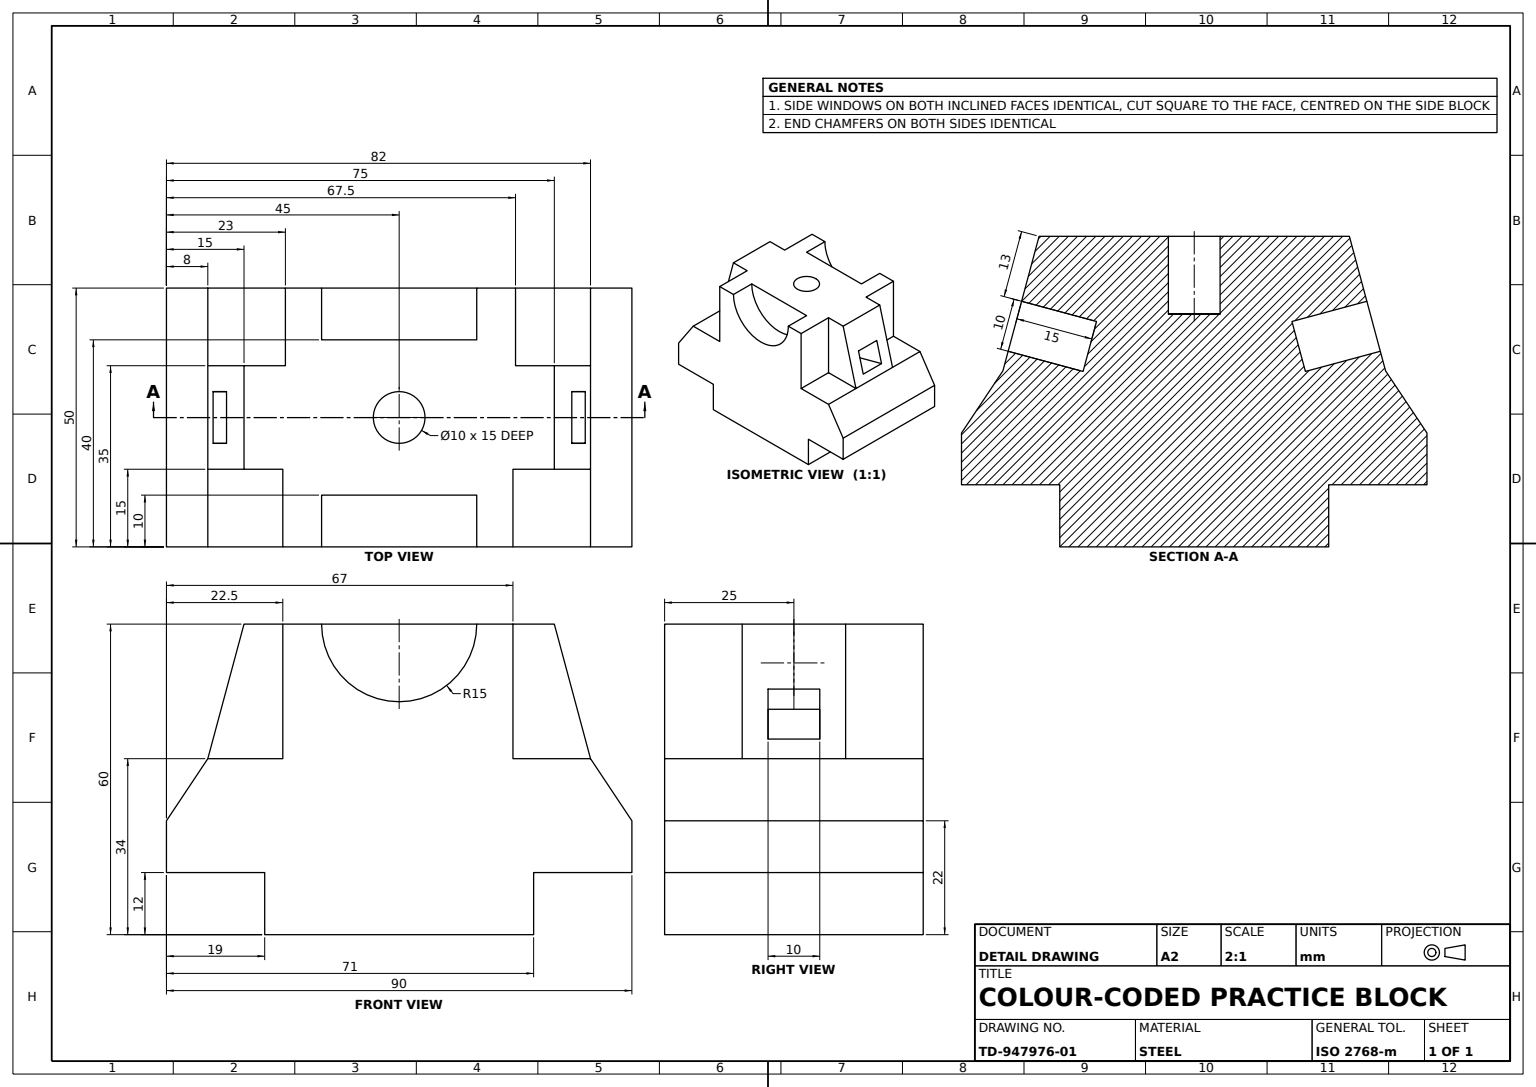
ISO-10303-21;
HEADER;
FILE_DESCRIPTION((''),'2;1');
FILE_NAME('','',(''),(''),'','','');
FILE_SCHEMA(('AUTOMOTIVE_DESIGN'));
ENDSEC;
DATA;
#1=APPLICATION_CONTEXT('');
#2=PRODUCT_CONTEXT('',#1,'mechanical');
#3=PRODUCT('','','',(#2));
#4=PRODUCT_DEFINITION_FORMATION('','',#3);
#5=PRODUCT_DEFINITION_CONTEXT('',#1,'design');
#6=PRODUCT_DEFINITION('','',#4,#5);
#7=PRODUCT_DEFINITION_SHAPE('','',#6);
#8=(LENGTH_UNIT()NAMED_UNIT(*)SI_UNIT(.MILLI.,.METRE.));
#9=(NAMED_UNIT(*)PLANE_ANGLE_UNIT()SI_UNIT($,.RADIAN.));
#10=(NAMED_UNIT(*)SI_UNIT($,.STERADIAN.)SOLID_ANGLE_UNIT());
#11=UNCERTAINTY_MEASURE_WITH_UNIT(LENGTH_MEASURE(1.E-05),#8,'distance_accuracy_value','');
#12=(GEOMETRIC_REPRESENTATION_CONTEXT(3)GLOBAL_UNCERTAINTY_ASSIGNED_CONTEXT((#11))GLOBAL_UNIT_ASSIGNED_CONTEXT((#8,#9,#10))REPRESENTATION_CONTEXT('',''));
#13=CARTESIAN_POINT('',(11.,60.,50.));
#14=VERTEX_POINT('',#13);
#15=CARTESIAN_POINT('',(41.,60.,50.));
#16=VERTEX_POINT('',#15);
#17=CARTESIAN_POINT('',(26.,60.,50.));
#18=DIRECTION('',(0.,0.,1.));
#19=DIRECTION('',(1.,0.,0.));
#20=AXIS2_PLACEMENT_3D('',#17,#18,#19);
#21=CIRCLE('',#20,15.);
#22=EDGE_CURVE('',#14,#16,#21,.T.);
#23=ORIENTED_EDGE('',*,*,#22,.F.);
#24=CARTESIAN_POINT('',(3.5,60.,50.));
#25=VERTEX_POINT('',#24);
#26=CARTESIAN_POINT('',(4.,60.,50.));
#27=DIRECTION('',(-1.,0.,0.));
#28=VECTOR('',#27,1000.);
#29=LINE('',#26,#28);
#30=EDGE_CURVE('',#14,#25,#29,.T.);
#31=ORIENTED_EDGE('',*,*,#30,.T.);
#32=CARTESIAN_POINT('',(3.5,34.,50.));
#33=VERTEX_POINT('',#32);
#34=DIRECTION('',(0.,1.,0.));
#35=VECTOR('',#34,1000.);
#36=LINE('',#24,#35);
#37=EDGE_CURVE('',#33,#25,#36,.T.);
#38=ORIENTED_EDGE('',*,*,#37,.F.);
#39=CARTESIAN_POINT('',(-11.,34.,50.));
#40=VERTEX_POINT('',#39);
#41=VECTOR('',#19,1000.);
#42=LINE('',#32,#41);
#43=EDGE_CURVE('',#40,#33,#42,.T.);
#44=ORIENTED_EDGE('',*,*,#43,.F.);
#45=CARTESIAN_POINT('',(-19.,22.,50.));
#46=VERTEX_POINT('',#45);
#47=DIRECTION('',(-0.554700196,-0.832050294,0.));
#48=VECTOR('',#47,1000.);
#49=LINE('',#39,#48);
#50=EDGE_CURVE('',#40,#46,#49,.T.);
#51=ORIENTED_EDGE('',*,*,#50,.T.);
#52=CARTESIAN_POINT('',(-19.,12.,50.));
#53=VERTEX_POINT('',#52);
#54=DIRECTION('',(0.,-1.,0.));
#55=VECTOR('',#54,1000.);
#56=LINE('',#52,#55);
#57=EDGE_CURVE('',#46,#53,#56,.T.);
#58=ORIENTED_EDGE('',*,*,#57,.T.);
#59=CARTESIAN_POINT('',(0.,12.,50.));
#60=VERTEX_POINT('',#59);
#61=LINE('',#59,#41);
#62=EDGE_CURVE('',#53,#60,#61,.T.);
#63=ORIENTED_EDGE('',*,*,#62,.T.);
#64=CARTESIAN_POINT('',(0.,0.,50.));
#65=VERTEX_POINT('',#64);
#66=LINE('',#64,#55);
#67=EDGE_CURVE('',#60,#65,#66,.T.);
#68=ORIENTED_EDGE('',*,*,#67,.T.);
#69=CARTESIAN_POINT('',(52.,0.,50.));
#70=VERTEX_POINT('',#69);
#71=LINE('',#64,#41);
#72=EDGE_CURVE('',#65,#70,#71,.T.);
#73=ORIENTED_EDGE('',*,*,#72,.T.);
#74=CARTESIAN_POINT('',(52.,12.,50.));
#75=VERTEX_POINT('',#74);
#76=LINE('',#69,#35);
#77=EDGE_CURVE('',#70,#75,#76,.T.);
#78=ORIENTED_EDGE('',*,*,#77,.T.);
#79=CARTESIAN_POINT('',(71.,12.,50.));
#80=VERTEX_POINT('',#79);
#81=LINE('',#74,#41);
#82=EDGE_CURVE('',#75,#80,#81,.T.);
#83=ORIENTED_EDGE('',*,*,#82,.T.);
#84=CARTESIAN_POINT('',(71.,22.,50.));
#85=VERTEX_POINT('',#84);
#86=LINE('',#79,#35);
#87=EDGE_CURVE('',#80,#85,#86,.T.);
#88=ORIENTED_EDGE('',*,*,#87,.T.);
#89=CARTESIAN_POINT('',(63.,34.,50.));
#90=VERTEX_POINT('',#89);
#91=DIRECTION('',(-0.554700196,0.832050294,0.));
#92=VECTOR('',#91,1000.);
#93=LINE('',#89,#92);
#94=EDGE_CURVE('',#85,#90,#93,.T.);
#95=ORIENTED_EDGE('',*,*,#94,.T.);
#96=CARTESIAN_POINT('',(48.,34.,50.));
#97=VERTEX_POINT('',#96);
#98=LINE('',#96,#28);
#99=EDGE_CURVE('',#90,#97,#98,.T.);
#100=ORIENTED_EDGE('',*,*,#99,.T.);
#101=CARTESIAN_POINT('',(48.,60.,50.));
#102=VERTEX_POINT('',#101);
#103=LINE('',#96,#35);
#104=EDGE_CURVE('',#97,#102,#103,.T.);
#105=ORIENTED_EDGE('',*,*,#104,.T.);
#106=EDGE_CURVE('',#102,#16,#29,.T.);
#107=ORIENTED_EDGE('',*,*,#106,.T.);
#108=EDGE_LOOP('',(#23,#31,#38,#44,#51,#58,#63,#68,#73,#78,#83,#88,#95,#100,#105,#107));
#109=FACE_OUTER_BOUND('',#108,.T.);
#110=AXIS2_PLACEMENT_3D('',#64,#18,#19);
#111=PLANE('',#110);
#112=ADVANCED_FACE('',(#109),#111,.T.);
#113=CARTESIAN_POINT('',(48.5,34.,0.));
#114=VERTEX_POINT('',#113);
#115=CARTESIAN_POINT('',(48.5,60.,0.));
#116=VERTEX_POINT('',#115);
#117=LINE('',#115,#35);
#118=EDGE_CURVE('',#114,#116,#117,.T.);
#119=ORIENTED_EDGE('',*,*,#118,.T.);
#120=CARTESIAN_POINT('',(48.5,60.,15.));
#121=VERTEX_POINT('',#120);
#122=CARTESIAN_POINT('',(48.5,60.,20.));
#123=DIRECTION('',(0.,0.,-1.));
#124=VECTOR('',#123,1000.);
#125=LINE('',#122,#124);
#126=EDGE_CURVE('',#121,#116,#125,.T.);
#127=ORIENTED_EDGE('',*,*,#126,.F.);
#128=CARTESIAN_POINT('',(48.5,34.,15.));
#129=VERTEX_POINT('',#128);
#130=LINE('',#128,#35);
#131=EDGE_CURVE('',#129,#121,#130,.T.);
#132=ORIENTED_EDGE('',*,*,#131,.F.);
#133=CARTESIAN_POINT('',(48.5,34.,20.));
#134=LINE('',#133,#124);
#135=EDGE_CURVE('',#129,#114,#134,.T.);
#136=ORIENTED_EDGE('',*,*,#135,.T.);
#137=EDGE_LOOP('',(#119,#127,#132,#136));
#138=FACE_OUTER_BOUND('',#137,.T.);
#139=AXIS2_PLACEMENT_3D('',#122,#27,#18);
#140=PLANE('',#139);
#141=ADVANCED_FACE('',(#138),#140,.F.);
#142=CARTESIAN_POINT('',(26.,45.,20.));
#143=VERTEX_POINT('',#142);
#144=CARTESIAN_POINT('',(26.,60.,20.));
#145=VERTEX_POINT('',#144);
#146=LINE('',#142,#35);
#147=EDGE_CURVE('',#143,#145,#146,.T.);
#148=ORIENTED_EDGE('',*,*,#147,.F.);
#149=CARTESIAN_POINT('',(26.,45.,30.));
#150=VERTEX_POINT('',#149);
#151=CARTESIAN_POINT('',(26.,45.,25.));
#152=AXIS2_PLACEMENT_3D('',#151,#34,#18);
#153=CIRCLE('',#152,5.);
#154=EDGE_CURVE('',#150,#143,#153,.T.);
#155=ORIENTED_EDGE('',*,*,#154,.F.);
#156=CARTESIAN_POINT('',(26.,60.,30.));
#157=VERTEX_POINT('',#156);
#158=LINE('',#149,#35);
#159=EDGE_CURVE('',#150,#157,#158,.T.);
#160=ORIENTED_EDGE('',*,*,#159,.T.);
#161=CARTESIAN_POINT('',(26.,60.,25.));
#162=AXIS2_PLACEMENT_3D('',#161,#34,#18);
#163=CIRCLE('',#162,5.);
#164=EDGE_CURVE('',#157,#145,#163,.T.);
#165=ORIENTED_EDGE('',*,*,#164,.T.);
#166=EDGE_LOOP('',(#148,#155,#160,#165));
#167=FACE_OUTER_BOUND('',#166,.T.);
#168=CYLINDRICAL_SURFACE('',#152,5.);
#169=ADVANCED_FACE('',(#167),#168,.F.);
#170=CARTESIAN_POINT('',(11.,60.,0.));
#171=VERTEX_POINT('',#170);
#172=CARTESIAN_POINT('',(4.,60.,0.));
#173=VERTEX_POINT('',#172);
#174=LINE('',#172,#28);
#175=EDGE_CURVE('',#171,#173,#174,.T.);
#176=ORIENTED_EDGE('',*,*,#175,.T.);
#177=CARTESIAN_POINT('',(4.,60.,15.));
#178=VERTEX_POINT('',#177);
#179=LINE('',#26,#124);
#180=EDGE_CURVE('',#178,#173,#179,.T.);
#181=ORIENTED_EDGE('',*,*,#180,.F.);
#182=CARTESIAN_POINT('',(-4.,60.,15.));
#183=VERTEX_POINT('',#182);
#184=LINE('',#177,#28);
#185=EDGE_CURVE('',#178,#183,#184,.T.);
#186=ORIENTED_EDGE('',*,*,#185,.T.);
#187=CARTESIAN_POINT('',(-4.,60.,35.));
#188=VERTEX_POINT('',#187);
#189=VECTOR('',#18,1000.);
#190=LINE('',#182,#189);
#191=EDGE_CURVE('',#183,#188,#190,.T.);
#192=ORIENTED_EDGE('',*,*,#191,.T.);
#193=CARTESIAN_POINT('',(3.5,60.,35.));
#194=VERTEX_POINT('',#193);
#195=LINE('',#187,#28);
#196=EDGE_CURVE('',#194,#188,#195,.T.);
#197=ORIENTED_EDGE('',*,*,#196,.F.);
#198=LINE('',#193,#189);
#199=EDGE_CURVE('',#194,#25,#198,.T.);
#200=ORIENTED_EDGE('',*,*,#199,.T.);
#201=ORIENTED_EDGE('',*,*,#30,.F.);
#202=CARTESIAN_POINT('',(11.,60.,40.));
#203=VERTEX_POINT('',#202);
#204=LINE('',#202,#189);
#205=EDGE_CURVE('',#203,#14,#204,.T.);
#206=ORIENTED_EDGE('',*,*,#205,.F.);
#207=CARTESIAN_POINT('',(41.,60.,40.));
#208=VERTEX_POINT('',#207);
#209=LINE('',#202,#28);
#210=EDGE_CURVE('',#208,#203,#209,.T.);
#211=ORIENTED_EDGE('',*,*,#210,.F.);
#212=LINE('',#207,#189);
#213=EDGE_CURVE('',#208,#16,#212,.T.);
#214=ORIENTED_EDGE('',*,*,#213,.T.);
#215=ORIENTED_EDGE('',*,*,#106,.F.);
#216=CARTESIAN_POINT('',(48.,60.,35.));
#217=VERTEX_POINT('',#216);
#218=LINE('',#101,#124);
#219=EDGE_CURVE('',#102,#217,#218,.T.);
#220=ORIENTED_EDGE('',*,*,#219,.T.);
#221=CARTESIAN_POINT('',(56.,60.,35.));
#222=VERTEX_POINT('',#221);
#223=LINE('',#216,#28);
#224=EDGE_CURVE('',#222,#217,#223,.T.);
#225=ORIENTED_EDGE('',*,*,#224,.F.);
#226=CARTESIAN_POINT('',(56.,60.,15.));
#227=VERTEX_POINT('',#226);
#228=CARTESIAN_POINT('',(56.,60.,30.));
#229=LINE('',#228,#124);
#230=EDGE_CURVE('',#222,#227,#229,.T.);
#231=ORIENTED_EDGE('',*,*,#230,.T.);
#232=LINE('',#120,#41);
#233=EDGE_CURVE('',#121,#227,#232,.T.);
#234=ORIENTED_EDGE('',*,*,#233,.F.);
#235=ORIENTED_EDGE('',*,*,#126,.T.);
#236=CARTESIAN_POINT('',(41.,60.,0.));
#237=VERTEX_POINT('',#236);
#238=EDGE_CURVE('',#116,#237,#174,.T.);
#239=ORIENTED_EDGE('',*,*,#238,.T.);
#240=CARTESIAN_POINT('',(41.,60.,10.));
#241=VERTEX_POINT('',#240);
#242=LINE('',#240,#124);
#243=EDGE_CURVE('',#241,#237,#242,.T.);
#244=ORIENTED_EDGE('',*,*,#243,.F.);
#245=CARTESIAN_POINT('',(11.,60.,10.));
#246=VERTEX_POINT('',#245);
#247=LINE('',#240,#41);
#248=EDGE_CURVE('',#246,#241,#247,.T.);
#249=ORIENTED_EDGE('',*,*,#248,.F.);
#250=LINE('',#245,#124);
#251=EDGE_CURVE('',#246,#171,#250,.T.);
#252=ORIENTED_EDGE('',*,*,#251,.T.);
#253=EDGE_LOOP('',(#176,#181,#186,#192,#197,#200,#201,#206,#211,#214,#215,#220,#225,#231,#234,#235,#239,#244,#249,#252));
#254=FACE_OUTER_BOUND('',#253,.T.);
#255=EDGE_CURVE('',#145,#157,#163,.T.);
#256=ORIENTED_EDGE('',*,*,#255,.F.);
#257=ORIENTED_EDGE('',*,*,#164,.F.);
#258=EDGE_LOOP('',(#256,#257));
#259=FACE_BOUND('',#258,.T.);
#260=AXIS2_PLACEMENT_3D('',#26,#54,#123);
#261=PLANE('',#260);
#262=ADVANCED_FACE('',(#254,#259),#261,.F.);
#263=ORIENTED_EDGE('',*,*,#37,.T.);
#264=ORIENTED_EDGE('',*,*,#199,.F.);
#265=CARTESIAN_POINT('',(3.5,34.,35.));
#266=VERTEX_POINT('',#265);
#267=LINE('',#193,#35);
#268=EDGE_CURVE('',#266,#194,#267,.T.);
#269=ORIENTED_EDGE('',*,*,#268,.F.);
#270=LINE('',#265,#189);
#271=EDGE_CURVE('',#266,#33,#270,.T.);
#272=ORIENTED_EDGE('',*,*,#271,.T.);
#273=EDGE_LOOP('',(#263,#264,#269,#272));
#274=FACE_OUTER_BOUND('',#273,.T.);
#275=AXIS2_PLACEMENT_3D('',#193,#19,#123);
#276=PLANE('',#275);
#277=ADVANCED_FACE('',(#274),#276,.F.);
#278=CARTESIAN_POINT('',(4.504846,33.891235,20.));
#279=VERTEX_POINT('',#278);
#280=CARTESIAN_POINT('',(4.504846,33.891235,30.));
#281=VERTEX_POINT('',#280);
#282=LINE('',#278,#189);
#283=EDGE_CURVE('',#279,#281,#282,.T.);
#284=ORIENTED_EDGE('',*,*,#283,.T.);
#285=CARTESIAN_POINT('',(7.104581,43.547393,30.));
#286=VERTEX_POINT('',#285);
#287=DIRECTION('',(0.259973473,0.965615759,0.));
#288=VECTOR('',#287,1000.);
#289=LINE('',#285,#288);
#290=EDGE_CURVE('',#281,#286,#289,.T.);
#291=ORIENTED_EDGE('',*,*,#290,.T.);
#292=CARTESIAN_POINT('',(7.104581,43.547393,20.));
#293=VERTEX_POINT('',#292);
#294=LINE('',#292,#124);
#295=EDGE_CURVE('',#286,#293,#294,.T.);
#296=ORIENTED_EDGE('',*,*,#295,.T.);
#297=DIRECTION('',(-0.259973473,-0.965615759,0.));
#298=VECTOR('',#297,1000.);
#299=LINE('',#292,#298);
#300=EDGE_CURVE('',#293,#279,#299,.T.);
#301=ORIENTED_EDGE('',*,*,#300,.T.);
#302=EDGE_LOOP('',(#284,#291,#296,#301));
#303=FACE_OUTER_BOUND('',#302,.T.);
#304=CARTESIAN_POINT('',(-4.307488,1.159708,0.));
#305=DIRECTION('',(-0.965615759,0.259973473,0.));
#306=AXIS2_PLACEMENT_3D('',#304,#305,#297);
#307=PLANE('',#306);
#308=ADVANCED_FACE('',(#303),#307,.T.);
#309=CARTESIAN_POINT('',(4.,34.,15.));
#310=VERTEX_POINT('',#309);
#311=CARTESIAN_POINT('',(4.,34.,0.));
#312=VERTEX_POINT('',#311);
#313=CARTESIAN_POINT('',(4.,34.,50.));
#314=LINE('',#313,#124);
#315=EDGE_CURVE('',#310,#312,#314,.T.);
#316=ORIENTED_EDGE('',*,*,#315,.T.);
#317=CARTESIAN_POINT('',(-11.,34.,0.));
#318=VERTEX_POINT('',#317);
#319=LINE('',#311,#28);
#320=EDGE_CURVE('',#312,#318,#319,.T.);
#321=ORIENTED_EDGE('',*,*,#320,.T.);
#322=CARTESIAN_POINT('',(-11.,34.,15.));
#323=VERTEX_POINT('',#322);
#324=LINE('',#39,#124);
#325=EDGE_CURVE('',#323,#318,#324,.T.);
#326=ORIENTED_EDGE('',*,*,#325,.F.);
#327=LINE('',#309,#41);
#328=EDGE_CURVE('',#323,#310,#327,.T.);
#329=ORIENTED_EDGE('',*,*,#328,.T.);
#330=EDGE_LOOP('',(#316,#321,#326,#329));
#331=FACE_OUTER_BOUND('',#330,.T.);
#332=AXIS2_PLACEMENT_3D('',#313,#54,#123);
#333=PLANE('',#332);
#334=ADVANCED_FACE('',(#331),#333,.F.);
#335=CARTESIAN_POINT('',(47.495154,33.891235,20.));
#336=VERTEX_POINT('',#335);
#337=CARTESIAN_POINT('',(61.97939,37.790838,20.));
#338=VERTEX_POINT('',#337);
#339=DIRECTION('',(0.965615759,0.259973473,0.));
#340=VECTOR('',#339,1000.);
#341=LINE('',#335,#340);
#342=EDGE_CURVE('',#336,#338,#341,.T.);
#343=ORIENTED_EDGE('',*,*,#342,.F.);
#344=CARTESIAN_POINT('',(47.495154,33.891235,30.));
#345=VERTEX_POINT('',#344);
#346=LINE('',#344,#124);
#347=EDGE_CURVE('',#345,#336,#346,.T.);
#348=ORIENTED_EDGE('',*,*,#347,.F.);
#349=CARTESIAN_POINT('',(61.97939,37.790838,30.));
#350=VERTEX_POINT('',#349);
#351=LINE('',#344,#340);
#352=EDGE_CURVE('',#345,#350,#351,.T.);
#353=ORIENTED_EDGE('',*,*,#352,.T.);
#354=LINE('',#349,#124);
#355=EDGE_CURVE('',#350,#338,#354,.T.);
#356=ORIENTED_EDGE('',*,*,#355,.T.);
#357=EDGE_LOOP('',(#343,#348,#353,#356));
#358=FACE_OUTER_BOUND('',#357,.T.);
#359=DIRECTION('',(0.259973473,-0.965615759,0.));
#360=AXIS2_PLACEMENT_3D('',#344,#359,#339);
#361=PLANE('',#360);
#362=ADVANCED_FACE('',(#358),#361,.F.);
#363=ORIENTED_EDGE('',*,*,#57,.F.);
#364=CARTESIAN_POINT('',(-19.,22.,0.));
#365=VERTEX_POINT('',#364);
#366=LINE('',#45,#124);
#367=EDGE_CURVE('',#46,#365,#366,.T.);
#368=ORIENTED_EDGE('',*,*,#367,.T.);
#369=CARTESIAN_POINT('',(-19.,12.,0.));
#370=VERTEX_POINT('',#369);
#371=LINE('',#369,#55);
#372=EDGE_CURVE('',#365,#370,#371,.T.);
#373=ORIENTED_EDGE('',*,*,#372,.T.);
#374=LINE('',#52,#124);
#375=EDGE_CURVE('',#53,#370,#374,.T.);
#376=ORIENTED_EDGE('',*,*,#375,.F.);
#377=EDGE_LOOP('',(#363,#368,#373,#376));
#378=FACE_OUTER_BOUND('',#377,.T.);
#379=AXIS2_PLACEMENT_3D('',#52,#19,#123);
#380=PLANE('',#379);
#381=ADVANCED_FACE('',(#378),#380,.F.);
#382=LINE('',#182,#298);
#383=EDGE_CURVE('',#183,#323,#382,.T.);
#384=ORIENTED_EDGE('',*,*,#383,.F.);
#385=ORIENTED_EDGE('',*,*,#185,.F.);
#386=LINE('',#177,#35);
#387=EDGE_CURVE('',#310,#178,#386,.T.);
#388=ORIENTED_EDGE('',*,*,#387,.F.);
#389=ORIENTED_EDGE('',*,*,#328,.F.);
#390=EDGE_LOOP('',(#384,#385,#388,#389));
#391=FACE_OUTER_BOUND('',#390,.T.);
#392=CARTESIAN_POINT('',(0.,0.,15.));
#393=AXIS2_PLACEMENT_3D('',#392,#18,#19);
#394=PLANE('',#393);
#395=ADVANCED_FACE('',(#391),#394,.F.);
#396=ORIENTED_EDGE('',*,*,#180,.T.);
#397=LINE('',#311,#55);
#398=EDGE_CURVE('',#173,#312,#397,.T.);
#399=ORIENTED_EDGE('',*,*,#398,.T.);
#400=ORIENTED_EDGE('',*,*,#315,.F.);
#401=ORIENTED_EDGE('',*,*,#387,.T.);
#402=EDGE_LOOP('',(#396,#399,#400,#401));
#403=FACE_OUTER_BOUND('',#402,.T.);
#404=AXIS2_PLACEMENT_3D('',#313,#19,#123);
#405=PLANE('',#404);
#406=ADVANCED_FACE('',(#403),#405,.F.);
#407=ORIENTED_EDGE('',*,*,#210,.T.);
#408=CARTESIAN_POINT('',(26.,60.,40.));
#409=AXIS2_PLACEMENT_3D('',#408,#18,#19);
#410=CIRCLE('',#409,15.);
#411=EDGE_CURVE('',#203,#208,#410,.T.);
#412=ORIENTED_EDGE('',*,*,#411,.T.);
#413=EDGE_LOOP('',(#407,#412));
#414=FACE_OUTER_BOUND('',#413,.T.);
#415=PLANE('',#409);
#416=ADVANCED_FACE('',(#414),#415,.T.);
#417=CARTESIAN_POINT('',(-7.379655,47.446995,20.));
#418=VERTEX_POINT('',#417);
#419=VECTOR('',#305,1000.);
#420=LINE('',#292,#419);
#421=EDGE_CURVE('',#293,#418,#420,.T.);
#422=ORIENTED_EDGE('',*,*,#421,.T.);
#423=CARTESIAN_POINT('',(-9.97939,37.790838,20.));
#424=VERTEX_POINT('',#423);
#425=LINE('',#417,#298);
#426=EDGE_CURVE('',#418,#424,#425,.T.);
#427=ORIENTED_EDGE('',*,*,#426,.T.);
#428=LINE('',#278,#419);
#429=EDGE_CURVE('',#279,#424,#428,.T.);
#430=ORIENTED_EDGE('',*,*,#429,.F.);
#431=ORIENTED_EDGE('',*,*,#300,.F.);
#432=EDGE_LOOP('',(#422,#427,#430,#431));
#433=FACE_OUTER_BOUND('',#432,.T.);
#434=AXIS2_PLACEMENT_3D('',#292,#123,#27);
#435=PLANE('',#434);
#436=ADVANCED_FACE('',(#433),#435,.F.);
#437=CARTESIAN_POINT('',(48.,34.,35.));
#438=VERTEX_POINT('',#437);
#439=CARTESIAN_POINT('',(63.,34.,35.));
#440=VERTEX_POINT('',#439);
#441=LINE('',#439,#41);
#442=EDGE_CURVE('',#438,#440,#441,.T.);
#443=ORIENTED_EDGE('',*,*,#442,.T.);
#444=DIRECTION('',(-0.259973473,0.965615759,0.));
#445=VECTOR('',#444,1000.);
#446=LINE('',#221,#445);
#447=EDGE_CURVE('',#440,#222,#446,.T.);
#448=ORIENTED_EDGE('',*,*,#447,.T.);
#449=ORIENTED_EDGE('',*,*,#224,.T.);
#450=LINE('',#437,#55);
#451=EDGE_CURVE('',#217,#438,#450,.T.);
#452=ORIENTED_EDGE('',*,*,#451,.T.);
#453=EDGE_LOOP('',(#443,#448,#449,#452));
#454=FACE_OUTER_BOUND('',#453,.T.);
#455=CARTESIAN_POINT('',(0.,0.,35.));
#456=AXIS2_PLACEMENT_3D('',#455,#123,#27);
#457=PLANE('',#456);
#458=ADVANCED_FACE('',(#454),#457,.F.);
#459=CARTESIAN_POINT('',(-9.97939,37.790838,30.));
#460=VERTEX_POINT('',#459);
#461=CARTESIAN_POINT('',(-7.379655,47.446995,30.));
#462=VERTEX_POINT('',#461);
#463=LINE('',#461,#288);
#464=EDGE_CURVE('',#460,#462,#463,.T.);
#465=ORIENTED_EDGE('',*,*,#464,.T.);
#466=LINE('',#285,#419);
#467=EDGE_CURVE('',#286,#462,#466,.T.);
#468=ORIENTED_EDGE('',*,*,#467,.F.);
#469=ORIENTED_EDGE('',*,*,#290,.F.);
#470=LINE('',#280,#419);
#471=EDGE_CURVE('',#281,#460,#470,.T.);
#472=ORIENTED_EDGE('',*,*,#471,.T.);
#473=EDGE_LOOP('',(#465,#468,#469,#472));
#474=FACE_OUTER_BOUND('',#473,.T.);
#475=AXIS2_PLACEMENT_3D('',#285,#18,#54);
#476=PLANE('',#475);
#477=ADVANCED_FACE('',(#474),#476,.F.);
#478=CARTESIAN_POINT('',(52.,12.,0.));
#479=VERTEX_POINT('',#478);
#480=LINE('',#74,#124);
#481=EDGE_CURVE('',#75,#479,#480,.T.);
#482=ORIENTED_EDGE('',*,*,#481,.T.);
#483=CARTESIAN_POINT('',(71.,12.,0.));
#484=VERTEX_POINT('',#483);
#485=LINE('',#478,#41);
#486=EDGE_CURVE('',#479,#484,#485,.T.);
#487=ORIENTED_EDGE('',*,*,#486,.T.);
#488=LINE('',#79,#124);
#489=EDGE_CURVE('',#80,#484,#488,.T.);
#490=ORIENTED_EDGE('',*,*,#489,.F.);
#491=ORIENTED_EDGE('',*,*,#82,.F.);
#492=EDGE_LOOP('',(#482,#487,#490,#491));
#493=FACE_OUTER_BOUND('',#492,.T.);
#494=AXIS2_PLACEMENT_3D('',#74,#34,#18);
#495=PLANE('',#494);
#496=ADVANCED_FACE('',(#493),#495,.F.);
#497=EDGE_CURVE('',#143,#150,#153,.T.);
#498=ORIENTED_EDGE('',*,*,#497,.T.);
#499=ORIENTED_EDGE('',*,*,#154,.T.);
#500=EDGE_LOOP('',(#498,#499));
#501=FACE_OUTER_BOUND('',#500,.T.);
#502=PLANE('',#152);
#503=ADVANCED_FACE('',(#501),#502,.T.);
#504=ORIENTED_EDGE('',*,*,#243,.T.);
#505=CARTESIAN_POINT('',(26.,60.,0.));
#506=AXIS2_PLACEMENT_3D('',#505,#123,#27);
#507=CIRCLE('',#506,15.);
#508=EDGE_CURVE('',#237,#171,#507,.T.);
#509=ORIENTED_EDGE('',*,*,#508,.T.);
#510=ORIENTED_EDGE('',*,*,#251,.F.);
#511=CARTESIAN_POINT('',(26.,60.,10.));
#512=AXIS2_PLACEMENT_3D('',#511,#123,#27);
#513=CIRCLE('',#512,15.);
#514=EDGE_CURVE('',#241,#246,#513,.T.);
#515=ORIENTED_EDGE('',*,*,#514,.F.);
#516=EDGE_LOOP('',(#504,#509,#510,#515));
#517=FACE_OUTER_BOUND('',#516,.T.);
#518=CYLINDRICAL_SURFACE('',#512,15.);
#519=ADVANCED_FACE('',(#517),#518,.F.);
#520=ORIENTED_EDGE('',*,*,#367,.F.);
#521=ORIENTED_EDGE('',*,*,#50,.F.);
#522=CARTESIAN_POINT('',(-11.,34.,35.));
#523=VERTEX_POINT('',#522);
#524=EDGE_CURVE('',#40,#523,#324,.T.);
#525=ORIENTED_EDGE('',*,*,#524,.T.);
#526=EDGE_CURVE('',#523,#323,#324,.T.);
#527=ORIENTED_EDGE('',*,*,#526,.T.);
#528=ORIENTED_EDGE('',*,*,#325,.T.);
#529=LINE('',#317,#48);
#530=EDGE_CURVE('',#318,#365,#529,.T.);
#531=ORIENTED_EDGE('',*,*,#530,.T.);
#532=EDGE_LOOP('',(#520,#521,#525,#527,#528,#531));
#533=FACE_OUTER_BOUND('',#532,.T.);
#534=DIRECTION('',(0.832050294,-0.554700196,0.));
#535=DIRECTION('',(0.554700196,0.832050294,0.));
#536=AXIS2_PLACEMENT_3D('',#39,#534,#535);
#537=PLANE('',#536);
#538=ADVANCED_FACE('',(#533),#537,.F.);
#539=ORIENTED_EDGE('',*,*,#268,.T.);
#540=ORIENTED_EDGE('',*,*,#196,.T.);
#541=LINE('',#522,#298);
#542=EDGE_CURVE('',#188,#523,#541,.T.);
#543=ORIENTED_EDGE('',*,*,#542,.T.);
#544=LINE('',#265,#41);
#545=EDGE_CURVE('',#523,#266,#544,.T.);
#546=ORIENTED_EDGE('',*,*,#545,.T.);
#547=EDGE_LOOP('',(#539,#540,#543,#546));
#548=FACE_OUTER_BOUND('',#547,.T.);
#549=ADVANCED_FACE('',(#548),#457,.F.);
#550=CARTESIAN_POINT('',(44.895419,43.547393,20.));
#551=VERTEX_POINT('',#550);
#552=LINE('',#550,#445);
#553=EDGE_CURVE('',#336,#551,#552,.T.);
#554=ORIENTED_EDGE('',*,*,#553,.F.);
#555=ORIENTED_EDGE('',*,*,#342,.T.);
#556=CARTESIAN_POINT('',(59.379655,47.446995,20.));
#557=VERTEX_POINT('',#556);
#558=LINE('',#556,#445);
#559=EDGE_CURVE('',#338,#557,#558,.T.);
#560=ORIENTED_EDGE('',*,*,#559,.T.);
#561=LINE('',#550,#340);
#562=EDGE_CURVE('',#551,#557,#561,.T.);
#563=ORIENTED_EDGE('',*,*,#562,.F.);
#564=EDGE_LOOP('',(#554,#555,#560,#563));
#565=FACE_OUTER_BOUND('',#564,.T.);
#566=AXIS2_PLACEMENT_3D('',#550,#123,#34);
#567=PLANE('',#566);
#568=ADVANCED_FACE('',(#565),#567,.F.);
#569=ORIENTED_EDGE('',*,*,#451,.F.);
#570=ORIENTED_EDGE('',*,*,#219,.F.);
#571=ORIENTED_EDGE('',*,*,#104,.F.);
#572=LINE('',#96,#124);
#573=EDGE_CURVE('',#97,#438,#572,.T.);
#574=ORIENTED_EDGE('',*,*,#573,.T.);
#575=EDGE_LOOP('',(#569,#570,#571,#574));
#576=FACE_OUTER_BOUND('',#575,.T.);
#577=AXIS2_PLACEMENT_3D('',#96,#27,#18);
#578=PLANE('',#577);
#579=ADVANCED_FACE('',(#576),#578,.F.);
#580=CARTESIAN_POINT('',(44.895419,43.547393,30.));
#581=VERTEX_POINT('',#580);
#582=CARTESIAN_POINT('',(59.379655,47.446995,30.));
#583=VERTEX_POINT('',#582);
#584=LINE('',#580,#340);
#585=EDGE_CURVE('',#581,#583,#584,.T.);
#586=ORIENTED_EDGE('',*,*,#585,.F.);
#587=LINE('',#580,#189);
#588=EDGE_CURVE('',#551,#581,#587,.T.);
#589=ORIENTED_EDGE('',*,*,#588,.F.);
#590=ORIENTED_EDGE('',*,*,#562,.T.);
#591=LINE('',#582,#189);
#592=EDGE_CURVE('',#557,#583,#591,.T.);
#593=ORIENTED_EDGE('',*,*,#592,.T.);
#594=EDGE_LOOP('',(#586,#589,#590,#593));
#595=FACE_OUTER_BOUND('',#594,.T.);
#596=DIRECTION('',(-0.965615759,-0.259973473,0.));
#597=AXIS2_PLACEMENT_3D('',#580,#444,#596);
#598=PLANE('',#597);
#599=ADVANCED_FACE('',(#595),#598,.F.);
#600=ORIENTED_EDGE('',*,*,#497,.F.);
#601=ORIENTED_EDGE('',*,*,#147,.T.);
#602=ORIENTED_EDGE('',*,*,#255,.T.);
#603=ORIENTED_EDGE('',*,*,#159,.F.);
#604=EDGE_LOOP('',(#600,#601,#602,#603));
#605=FACE_OUTER_BOUND('',#604,.T.);
#606=ADVANCED_FACE('',(#605),#168,.F.);
#607=ORIENTED_EDGE('',*,*,#320,.F.);
#608=ORIENTED_EDGE('',*,*,#398,.F.);
#609=ORIENTED_EDGE('',*,*,#175,.F.);
#610=ORIENTED_EDGE('',*,*,#508,.F.);
#611=ORIENTED_EDGE('',*,*,#238,.F.);
#612=ORIENTED_EDGE('',*,*,#118,.F.);
#613=CARTESIAN_POINT('',(63.,34.,0.));
#614=VERTEX_POINT('',#613);
#615=LINE('',#113,#28);
#616=EDGE_CURVE('',#614,#114,#615,.T.);
#617=ORIENTED_EDGE('',*,*,#616,.F.);
#618=CARTESIAN_POINT('',(71.,22.,0.));
#619=VERTEX_POINT('',#618);
#620=LINE('',#613,#92);
#621=EDGE_CURVE('',#619,#614,#620,.T.);
#622=ORIENTED_EDGE('',*,*,#621,.F.);
#623=LINE('',#483,#35);
#624=EDGE_CURVE('',#484,#619,#623,.T.);
#625=ORIENTED_EDGE('',*,*,#624,.F.);
#626=ORIENTED_EDGE('',*,*,#486,.F.);
#627=CARTESIAN_POINT('',(52.,0.,0.));
#628=VERTEX_POINT('',#627);
#629=LINE('',#627,#35);
#630=EDGE_CURVE('',#628,#479,#629,.T.);
#631=ORIENTED_EDGE('',*,*,#630,.F.);
#632=CARTESIAN_POINT('',(0.,0.,0.));
#633=VERTEX_POINT('',#632);
#634=LINE('',#632,#41);
#635=EDGE_CURVE('',#633,#628,#634,.T.);
#636=ORIENTED_EDGE('',*,*,#635,.F.);
#637=CARTESIAN_POINT('',(0.,12.,0.));
#638=VERTEX_POINT('',#637);
#639=LINE('',#632,#55);
#640=EDGE_CURVE('',#638,#633,#639,.T.);
#641=ORIENTED_EDGE('',*,*,#640,.F.);
#642=LINE('',#637,#41);
#643=EDGE_CURVE('',#370,#638,#642,.T.);
#644=ORIENTED_EDGE('',*,*,#643,.F.);
#645=ORIENTED_EDGE('',*,*,#372,.F.);
#646=ORIENTED_EDGE('',*,*,#530,.F.);
#647=EDGE_LOOP('',(#607,#608,#609,#610,#611,#612,#617,#622,#625,#626,#631,#636,#641,#644,#645,#646));
#648=FACE_OUTER_BOUND('',#647,.T.);
#649=AXIS2_PLACEMENT_3D('',#632,#18,#19);
#650=PLANE('',#649);
#651=ADVANCED_FACE('',(#648),#650,.F.);
#652=VECTOR('',#359,1000.);
#653=LINE('',#580,#652);
#654=EDGE_CURVE('',#581,#345,#653,.T.);
#655=ORIENTED_EDGE('',*,*,#654,.F.);
#656=ORIENTED_EDGE('',*,*,#585,.T.);
#657=LINE('',#582,#652);
#658=EDGE_CURVE('',#583,#350,#657,.T.);
#659=ORIENTED_EDGE('',*,*,#658,.T.);
#660=ORIENTED_EDGE('',*,*,#352,.F.);
#661=EDGE_LOOP('',(#655,#656,#659,#660));
#662=FACE_OUTER_BOUND('',#661,.T.);
#663=AXIS2_PLACEMENT_3D('',#580,#18,#19);
#664=PLANE('',#663);
#665=ADVANCED_FACE('',(#662),#664,.F.);
#666=ORIENTED_EDGE('',*,*,#447,.F.);
#667=CARTESIAN_POINT('',(63.,34.,15.));
#668=VERTEX_POINT('',#667);
#669=CARTESIAN_POINT('',(63.,34.,30.));
#670=LINE('',#669,#124);
#671=EDGE_CURVE('',#440,#668,#670,.T.);
#672=ORIENTED_EDGE('',*,*,#671,.T.);
#673=LINE('',#226,#652);
#674=EDGE_CURVE('',#227,#668,#673,.T.);
#675=ORIENTED_EDGE('',*,*,#674,.F.);
#676=ORIENTED_EDGE('',*,*,#230,.F.);
#677=EDGE_LOOP('',(#666,#672,#675,#676));
#678=FACE_OUTER_BOUND('',#677,.T.);
#679=ORIENTED_EDGE('',*,*,#559,.F.);
#680=ORIENTED_EDGE('',*,*,#355,.F.);
#681=ORIENTED_EDGE('',*,*,#658,.F.);
#682=ORIENTED_EDGE('',*,*,#592,.F.);
#683=EDGE_LOOP('',(#679,#680,#681,#682));
#684=FACE_BOUND('',#683,.T.);
#685=AXIS2_PLACEMENT_3D('',#228,#339,#444);
#686=PLANE('',#685);
#687=ADVANCED_FACE('',(#678,#684),#686,.T.);
#688=ORIENTED_EDGE('',*,*,#43,.T.);
#689=ORIENTED_EDGE('',*,*,#271,.F.);
#690=ORIENTED_EDGE('',*,*,#545,.F.);
#691=ORIENTED_EDGE('',*,*,#524,.F.);
#692=EDGE_LOOP('',(#688,#689,#690,#691));
#693=FACE_OUTER_BOUND('',#692,.T.);
#694=AXIS2_PLACEMENT_3D('',#265,#54,#123);
#695=PLANE('',#694);
#696=ADVANCED_FACE('',(#693),#695,.F.);
#697=LINE('',#84,#124);
#698=EDGE_CURVE('',#85,#619,#697,.T.);
#699=ORIENTED_EDGE('',*,*,#698,.F.);
#700=ORIENTED_EDGE('',*,*,#87,.F.);
#701=ORIENTED_EDGE('',*,*,#489,.T.);
#702=ORIENTED_EDGE('',*,*,#624,.T.);
#703=EDGE_LOOP('',(#699,#700,#701,#702));
#704=FACE_OUTER_BOUND('',#703,.T.);
#705=AXIS2_PLACEMENT_3D('',#79,#27,#18);
#706=PLANE('',#705);
#707=ADVANCED_FACE('',(#704),#706,.F.);
#708=ORIENTED_EDGE('',*,*,#375,.T.);
#709=ORIENTED_EDGE('',*,*,#643,.T.);
#710=LINE('',#59,#124);
#711=EDGE_CURVE('',#60,#638,#710,.T.);
#712=ORIENTED_EDGE('',*,*,#711,.F.);
#713=ORIENTED_EDGE('',*,*,#62,.F.);
#714=EDGE_LOOP('',(#708,#709,#712,#713));
#715=FACE_OUTER_BOUND('',#714,.T.);
#716=AXIS2_PLACEMENT_3D('',#59,#34,#18);
#717=PLANE('',#716);
#718=ADVANCED_FACE('',(#715),#717,.F.);
#719=ORIENTED_EDGE('',*,*,#467,.T.);
#720=LINE('',#417,#124);
#721=EDGE_CURVE('',#462,#418,#720,.T.);
#722=ORIENTED_EDGE('',*,*,#721,.T.);
#723=ORIENTED_EDGE('',*,*,#421,.F.);
#724=ORIENTED_EDGE('',*,*,#295,.F.);
#725=EDGE_LOOP('',(#719,#722,#723,#724));
#726=FACE_OUTER_BOUND('',#725,.T.);
#727=AXIS2_PLACEMENT_3D('',#292,#287,#305);
#728=PLANE('',#727);
#729=ADVANCED_FACE('',(#726),#728,.F.);
#730=ORIENTED_EDGE('',*,*,#481,.F.);
#731=ORIENTED_EDGE('',*,*,#77,.F.);
#732=LINE('',#69,#124);
#733=EDGE_CURVE('',#70,#628,#732,.T.);
#734=ORIENTED_EDGE('',*,*,#733,.T.);
#735=ORIENTED_EDGE('',*,*,#630,.T.);
#736=EDGE_LOOP('',(#730,#731,#734,#735));
#737=FACE_OUTER_BOUND('',#736,.T.);
#738=AXIS2_PLACEMENT_3D('',#69,#27,#18);
#739=PLANE('',#738);
#740=ADVANCED_FACE('',(#737),#739,.F.);
#741=ORIENTED_EDGE('',*,*,#635,.T.);
#742=ORIENTED_EDGE('',*,*,#733,.F.);
#743=ORIENTED_EDGE('',*,*,#72,.F.);
#744=LINE('',#64,#124);
#745=EDGE_CURVE('',#65,#633,#744,.T.);
#746=ORIENTED_EDGE('',*,*,#745,.T.);
#747=EDGE_LOOP('',(#741,#742,#743,#746));
#748=FACE_OUTER_BOUND('',#747,.T.);
#749=AXIS2_PLACEMENT_3D('',#64,#34,#18);
#750=PLANE('',#749);
#751=ADVANCED_FACE('',(#748),#750,.F.);
#752=ORIENTED_EDGE('',*,*,#131,.T.);
#753=ORIENTED_EDGE('',*,*,#233,.T.);
#754=ORIENTED_EDGE('',*,*,#674,.T.);
#755=LINE('',#667,#28);
#756=EDGE_CURVE('',#668,#129,#755,.T.);
#757=ORIENTED_EDGE('',*,*,#756,.T.);
#758=EDGE_LOOP('',(#752,#753,#754,#757));
#759=FACE_OUTER_BOUND('',#758,.T.);
#760=AXIS2_PLACEMENT_3D('',#392,#123,#27);
#761=PLANE('',#760);
#762=ADVANCED_FACE('',(#759),#761,.T.);
#763=ORIENTED_EDGE('',*,*,#640,.T.);
#764=ORIENTED_EDGE('',*,*,#745,.F.);
#765=ORIENTED_EDGE('',*,*,#67,.F.);
#766=ORIENTED_EDGE('',*,*,#711,.T.);
#767=EDGE_LOOP('',(#763,#764,#765,#766));
#768=FACE_OUTER_BOUND('',#767,.T.);
#769=AXIS2_PLACEMENT_3D('',#64,#19,#123);
#770=PLANE('',#769);
#771=ADVANCED_FACE('',(#768),#770,.F.);
#772=ORIENTED_EDGE('',*,*,#135,.F.);
#773=ORIENTED_EDGE('',*,*,#756,.F.);
#774=CARTESIAN_POINT('',(63.,34.,20.));
#775=LINE('',#774,#124);
#776=EDGE_CURVE('',#668,#614,#775,.T.);
#777=ORIENTED_EDGE('',*,*,#776,.T.);
#778=ORIENTED_EDGE('',*,*,#616,.T.);
#779=EDGE_LOOP('',(#772,#773,#777,#778));
#780=FACE_OUTER_BOUND('',#779,.T.);
#781=AXIS2_PLACEMENT_3D('',#133,#54,#123);
#782=PLANE('',#781);
#783=ADVANCED_FACE('',(#780),#782,.F.);
#784=ORIENTED_EDGE('',*,*,#776,.F.);
#785=ORIENTED_EDGE('',*,*,#671,.F.);
#786=LINE('',#89,#124);
#787=EDGE_CURVE('',#90,#440,#786,.T.);
#788=ORIENTED_EDGE('',*,*,#787,.F.);
#789=ORIENTED_EDGE('',*,*,#94,.F.);
#790=ORIENTED_EDGE('',*,*,#698,.T.);
#791=ORIENTED_EDGE('',*,*,#621,.T.);
#792=EDGE_LOOP('',(#784,#785,#788,#789,#790,#791));
#793=FACE_OUTER_BOUND('',#792,.T.);
#794=DIRECTION('',(-0.832050294,-0.554700196,0.));
#795=DIRECTION('',(0.554700196,-0.832050294,0.));
#796=AXIS2_PLACEMENT_3D('',#89,#794,#795);
#797=PLANE('',#796);
#798=ADVANCED_FACE('',(#793),#797,.F.);
#799=ORIENTED_EDGE('',*,*,#347,.T.);
#800=ORIENTED_EDGE('',*,*,#553,.T.);
#801=ORIENTED_EDGE('',*,*,#588,.T.);
#802=ORIENTED_EDGE('',*,*,#654,.T.);
#803=EDGE_LOOP('',(#799,#800,#801,#802));
#804=FACE_OUTER_BOUND('',#803,.T.);
#805=CARTESIAN_POINT('',(52.793005,14.213501,0.));
#806=AXIS2_PLACEMENT_3D('',#805,#339,#444);
#807=PLANE('',#806);
#808=ADVANCED_FACE('',(#804),#807,.T.);
#809=ORIENTED_EDGE('',*,*,#542,.F.);
#810=ORIENTED_EDGE('',*,*,#191,.F.);
#811=ORIENTED_EDGE('',*,*,#383,.T.);
#812=ORIENTED_EDGE('',*,*,#526,.F.);
#813=EDGE_LOOP('',(#809,#810,#811,#812));
#814=FACE_OUTER_BOUND('',#813,.T.);
#815=ORIENTED_EDGE('',*,*,#464,.F.);
#816=LINE('',#423,#189);
#817=EDGE_CURVE('',#424,#460,#816,.T.);
#818=ORIENTED_EDGE('',*,*,#817,.F.);
#819=ORIENTED_EDGE('',*,*,#426,.F.);
#820=ORIENTED_EDGE('',*,*,#721,.F.);
#821=EDGE_LOOP('',(#815,#818,#819,#820));
#822=FACE_BOUND('',#821,.T.);
#823=AXIS2_PLACEMENT_3D('',#182,#305,#297);
#824=PLANE('',#823);
#825=ADVANCED_FACE('',(#814,#822),#824,.T.);
#826=ORIENTED_EDGE('',*,*,#283,.F.);
#827=ORIENTED_EDGE('',*,*,#429,.T.);
#828=ORIENTED_EDGE('',*,*,#817,.T.);
#829=ORIENTED_EDGE('',*,*,#471,.F.);
#830=EDGE_LOOP('',(#826,#827,#828,#829));
#831=FACE_OUTER_BOUND('',#830,.T.);
#832=DIRECTION('',(0.965615759,-0.259973473,0.));
#833=AXIS2_PLACEMENT_3D('',#278,#297,#832);
#834=PLANE('',#833);
#835=ADVANCED_FACE('',(#831),#834,.F.);
#836=ORIENTED_EDGE('',*,*,#213,.F.);
#837=ORIENTED_EDGE('',*,*,#411,.F.);
#838=ORIENTED_EDGE('',*,*,#205,.T.);
#839=ORIENTED_EDGE('',*,*,#22,.T.);
#840=EDGE_LOOP('',(#836,#837,#838,#839));
#841=FACE_OUTER_BOUND('',#840,.T.);
#842=CYLINDRICAL_SURFACE('',#409,15.);
#843=ADVANCED_FACE('',(#841),#842,.F.);
#844=ORIENTED_EDGE('',*,*,#787,.T.);
#845=ORIENTED_EDGE('',*,*,#442,.F.);
#846=ORIENTED_EDGE('',*,*,#573,.F.);
#847=ORIENTED_EDGE('',*,*,#99,.F.);
#848=EDGE_LOOP('',(#844,#845,#846,#847));
#849=FACE_OUTER_BOUND('',#848,.T.);
#850=AXIS2_PLACEMENT_3D('',#96,#54,#123);
#851=PLANE('',#850);
#852=ADVANCED_FACE('',(#849),#851,.F.);
#853=ORIENTED_EDGE('',*,*,#248,.T.);
#854=ORIENTED_EDGE('',*,*,#514,.T.);
#855=EDGE_LOOP('',(#853,#854));
#856=FACE_OUTER_BOUND('',#855,.T.);
#857=PLANE('',#512);
#858=ADVANCED_FACE('',(#856),#857,.T.);
#859=CLOSED_SHELL('',(#112,#141,#169,#262,#277,#308,#334,#362,#381,#395,#406,#416,#436,#458,#477,#496,#503,#519,#538,#549,#568,#579,#599,#606,#651,#665,#687,#696,#707,#718,#729,#740,#751,#762,#771,#783,#798,#808,#825,#835,#843,#852,#858));
#860=MANIFOLD_SOLID_BREP('',#859);
#861=ADVANCED_BREP_SHAPE_REPRESENTATION('',(#860),#12);
#862=SHAPE_DEFINITION_REPRESENTATION(#7,#861);
ENDSEC;
END-ISO-10303-21;
